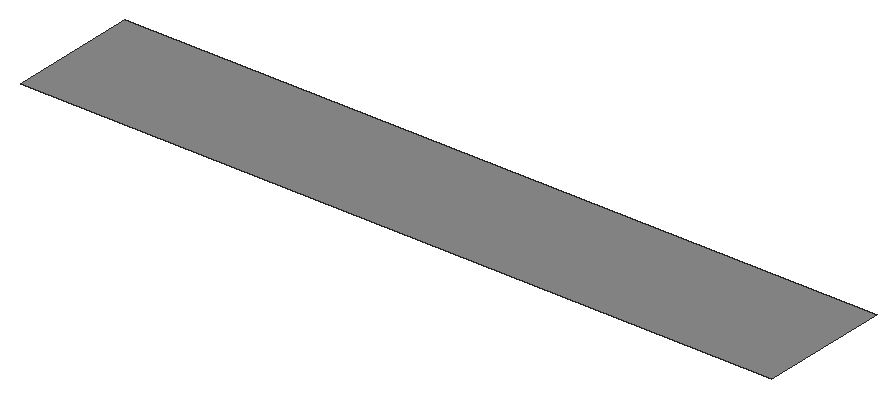
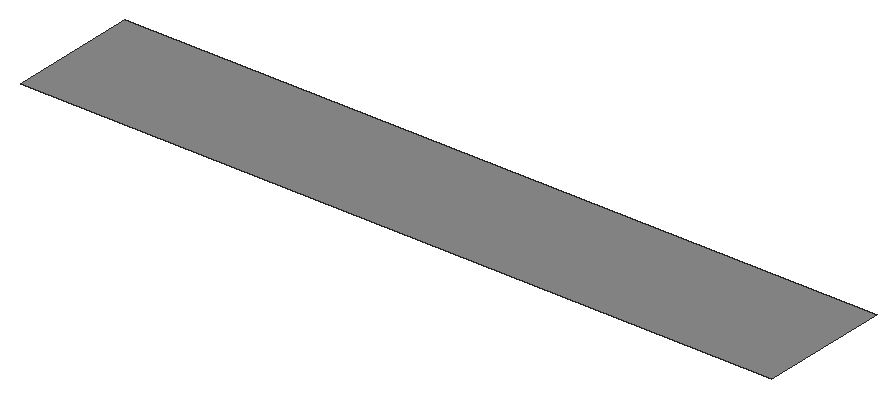
# SketchUp Ruby script. Lengths in inches.
U = 1.inch
M = Sketchup.active_model
def pt(a) = Geom::Point3d.new(a.map { |v| v * U })
def face(e, loops, mat)
  f = e.add_face(loops[0].map { |a| pt(a) })
  loops[1..].each { |l| e.add_face(l.map { |a| pt(a) }).erase! }
  f.material = f.back_material = mat if mat
  f
end
# faces: each face lists its corners as indices into pts; further lists are holes
def faces(e, pts, list, mat = nil) = list.each { |f| face(e, (f[0].is_a?(Array) ? f : [f]).map { |l| l.map { |i| pts[i] } }, mat) }
# xy, xz, yz: faces in a plane at the given z, y or x. An outline is a flat list of corners, or four numbers for a rectangle; further outlines are holes
def ring(l) = l.size == 4 ? [[l[0], l[1]], [l[2], l[1]], [l[2], l[3]], [l[0], l[3]]] : l.each_slice(2).to_a
def flat(e, list, mat, &to3) = list.each { |f| face(e, (f[0].is_a?(Array) ? f : [f]).map { |l| ring(l).map { |u, v| to3.(u, v) } }, mat) }
def xy(e, z, list, mat = nil) = flat(e, list, mat) { |x, y| [x, y, z] }
def xz(e, y, list, mat = nil) = flat(e, list, mat) { |x, z| [x, y, z] }
def yz(e, x, list, mat = nil) = flat(e, list, mat) { |y, z| [x, y, z] }
def lines(e, pts, list) = list.each { |a, b| e.add_line(pt(pts[a]), pt(pts[b])) }
# prism: a flat outline (further loops are holes) pulled along v
def prism(e, loops, v, mat = nil)
  f = face(e, loops, mat); d = Geom::Vector3d.new(v.map { |x| x * U })
  f.pushpull(f.normal.samedirection?(d) ? d.length : -d.length)
end
def box(e, o, s, mat = nil) = prism(e, [[o, [o[0] + s[0], o[1], o[2]], [o[0] + s[0], o[1] + s[1], o[2]], [o[0], o[1] + s[1], o[2]]]], [0, 0, s[2]], mat)
def at(x, y, z, deg = 0) = Geom::Transformation.translation(pt([x, y, z])) * Geom::Transformation.rotation(ORIGIN, Z_AXIS, deg.degrees)
def axes(o, x, y, z) = Geom::Transformation.new([*x, 0, *y, 0, *z, 0, *pt(o).to_a, 1])
def part(name) = M.definitions.add(name)
# library, detail: a bought-in or finely detailed component or shape, given as its bounding box
def library(name, o, s) = part(name).tap { |d| box(d.entities, o, s) }
def detail(e, o, s) = box(e.add_group.entities, o, s)
def put(e, d, t, mat = nil) = e.add_instance(d, t).tap { |i| i.material = mat if mat }
def group(e, t, mat = nil) = e.add_group.tap { |g| g.transformation = t; g.material = mat if mat }.entities
root = M.entities
M.materials.add("[Color M04]").color = [142, 142, 142]
xy(root,0,[[0,0,469.67,81.92]],"[Color M04]")
